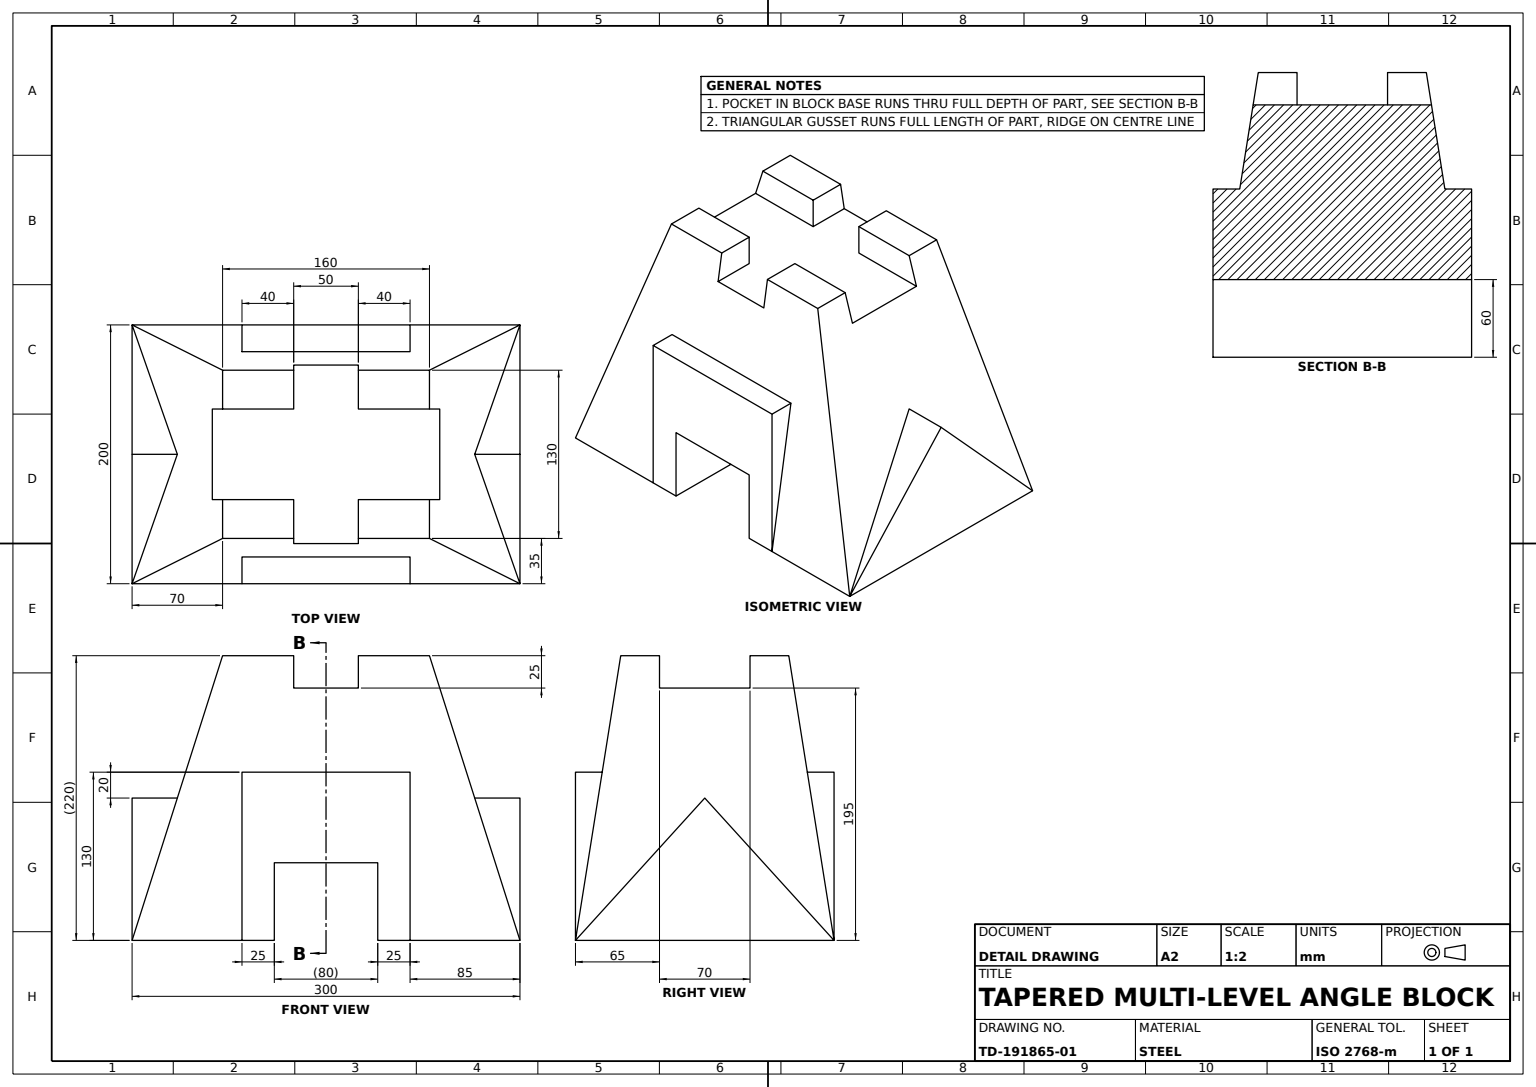
ISO-10303-21;
HEADER;
FILE_DESCRIPTION((''),'2;1');
FILE_NAME('','',(''),(''),'','','');
FILE_SCHEMA(('AUTOMOTIVE_DESIGN'));
ENDSEC;
DATA;
#1=APPLICATION_CONTEXT('');
#2=PRODUCT_CONTEXT('',#1,'mechanical');
#3=PRODUCT('','','',(#2));
#4=PRODUCT_DEFINITION_FORMATION('','',#3);
#5=PRODUCT_DEFINITION_CONTEXT('',#1,'design');
#6=PRODUCT_DEFINITION('','',#4,#5);
#7=PRODUCT_DEFINITION_SHAPE('','',#6);
#8=(LENGTH_UNIT()NAMED_UNIT(*)SI_UNIT(.MILLI.,.METRE.));
#9=(NAMED_UNIT(*)PLANE_ANGLE_UNIT()SI_UNIT($,.RADIAN.));
#10=(NAMED_UNIT(*)SI_UNIT($,.STERADIAN.)SOLID_ANGLE_UNIT());
#11=UNCERTAINTY_MEASURE_WITH_UNIT(LENGTH_MEASURE(0.005),#8,'distance_accuracy_value','');
#12=(GEOMETRIC_REPRESENTATION_CONTEXT(3)GLOBAL_UNCERTAINTY_ASSIGNED_CONTEXT((#11))GLOBAL_UNIT_ASSIGNED_CONTEXT((#8,#9,#10))REPRESENTATION_CONTEXT('',''));
#13=CARTESIAN_POINT('',(-100.,65.,130.));
#14=VERTEX_POINT('',#13);
#15=CARTESIAN_POINT('',(-100.,65.,0.));
#16=VERTEX_POINT('',#15);
#17=DIRECTION('',(0.,0.,-1.));
#18=VECTOR('',#17,1000.);
#19=LINE('',#13,#18);
#20=EDGE_CURVE('',#14,#16,#19,.T.);
#21=ORIENTED_EDGE('',*,*,#20,.T.);
#22=CARTESIAN_POINT('',(-100.,40.,0.));
#23=VERTEX_POINT('',#22);
#24=DIRECTION('',(0.,-1.,0.));
#25=VECTOR('',#24,1000.);
#26=LINE('',#15,#25);
#27=EDGE_CURVE('',#16,#23,#26,.T.);
#28=ORIENTED_EDGE('',*,*,#27,.T.);
#29=CARTESIAN_POINT('',(-100.,40.,60.));
#30=VERTEX_POINT('',#29);
#31=LINE('',#22,#18);
#32=EDGE_CURVE('',#30,#23,#31,.T.);
#33=ORIENTED_EDGE('',*,*,#32,.F.);
#34=CARTESIAN_POINT('',(-100.,-40.,60.));
#35=VERTEX_POINT('',#34);
#36=CARTESIAN_POINT('',(-100.,0.,60.));
#37=DIRECTION('',(0.,1.,0.));
#38=VECTOR('',#37,1000.);
#39=LINE('',#36,#38);
#40=EDGE_CURVE('',#35,#30,#39,.T.);
#41=ORIENTED_EDGE('',*,*,#40,.F.);
#42=CARTESIAN_POINT('',(-100.,-40.,0.));
#43=VERTEX_POINT('',#42);
#44=DIRECTION('',(0.,0.,1.));
#45=VECTOR('',#44,1000.);
#46=LINE('',#42,#45);
#47=EDGE_CURVE('',#43,#35,#46,.T.);
#48=ORIENTED_EDGE('',*,*,#47,.F.);
#49=CARTESIAN_POINT('',(-100.,-65.,0.));
#50=VERTEX_POINT('',#49);
#51=EDGE_CURVE('',#43,#50,#26,.T.);
#52=ORIENTED_EDGE('',*,*,#51,.T.);
#53=CARTESIAN_POINT('',(-100.,-65.,130.));
#54=VERTEX_POINT('',#53);
#55=LINE('',#49,#45);
#56=EDGE_CURVE('',#50,#54,#55,.T.);
#57=ORIENTED_EDGE('',*,*,#56,.T.);
#58=LINE('',#53,#38);
#59=EDGE_CURVE('',#54,#14,#58,.T.);
#60=ORIENTED_EDGE('',*,*,#59,.T.);
#61=EDGE_LOOP('',(#21,#28,#33,#41,#48,#52,#57,#60));
#62=FACE_BOUND('',#61,.T.);
#63=CARTESIAN_POINT('',(-100.,0.,0.));
#64=DIRECTION('',(-1.,0.,0.));
#65=AXIS2_PLACEMENT_3D('',#63,#64,#44);
#66=PLANE('',#65);
#67=ADVANCED_FACE('',(#62),#66,.T.);
#68=CARTESIAN_POINT('',(100.,150.,0.));
#69=VERTEX_POINT('',#68);
#70=CARTESIAN_POINT('',(0.,150.,110.));
#71=VERTEX_POINT('',#70);
#72=DIRECTION('',(-0.672672794,0.,0.739940073));
#73=VECTOR('',#72,1000.);
#74=LINE('',#68,#73);
#75=EDGE_CURVE('',#69,#71,#74,.T.);
#76=ORIENTED_EDGE('',*,*,#75,.F.);
#77=CARTESIAN_POINT('',(-100.,150.,0.));
#78=VERTEX_POINT('',#77);
#79=VECTOR('',#64,1000.);
#80=LINE('',#68,#79);
#81=EDGE_CURVE('',#69,#78,#80,.T.);
#82=ORIENTED_EDGE('',*,*,#81,.T.);
#83=DIRECTION('',(-0.672672794,0.,-0.739940073));
#84=VECTOR('',#83,1000.);
#85=LINE('',#70,#84);
#86=EDGE_CURVE('',#71,#78,#85,.T.);
#87=ORIENTED_EDGE('',*,*,#86,.F.);
#88=EDGE_LOOP('',(#76,#82,#87));
#89=FACE_BOUND('',#88,.T.);
#90=CARTESIAN_POINT('',(0.,150.,0.));
#91=AXIS2_PLACEMENT_3D('',#90,#24,#17);
#92=PLANE('',#91);
#93=ADVANCED_FACE('',(#89),#92,.F.);
#94=CARTESIAN_POINT('',(35.,-25.,195.));
#95=VERTEX_POINT('',#94);
#96=CARTESIAN_POINT('',(35.,-25.,220.));
#97=VERTEX_POINT('',#96);
#98=CARTESIAN_POINT('',(35.,-25.,265.));
#99=LINE('',#98,#18);
#100=EDGE_CURVE('',#95,#97,#99,.F.);
#101=ORIENTED_EDGE('',*,*,#100,.F.);
#102=CARTESIAN_POINT('',(35.,-87.954545,195.));
#103=VERTEX_POINT('',#102);
#104=CARTESIAN_POINT('',(35.,-220.,195.));
#105=LINE('',#104,#38);
#106=EDGE_CURVE('',#103,#95,#105,.T.);
#107=ORIENTED_EDGE('',*,*,#106,.F.);
#108=CARTESIAN_POINT('',(35.,-80.,220.));
#109=VERTEX_POINT('',#108);
#110=DIRECTION('',(0.,-0.303203657,-0.95292578));
#111=VECTOR('',#110,1000.);
#112=LINE('',#108,#111);
#113=EDGE_CURVE('',#109,#103,#112,.T.);
#114=ORIENTED_EDGE('',*,*,#113,.F.);
#115=CARTESIAN_POINT('',(35.,-220.,220.));
#116=LINE('',#115,#38);
#117=EDGE_CURVE('',#109,#97,#116,.T.);
#118=ORIENTED_EDGE('',*,*,#117,.T.);
#119=EDGE_LOOP('',(#101,#107,#114,#118));
#120=FACE_BOUND('',#119,.T.);
#121=DIRECTION('',(1.,0.,0.));
#122=AXIS2_PLACEMENT_3D('',#115,#121,#17);
#123=PLANE('',#122);
#124=ADVANCED_FACE('',(#120),#123,.F.);
#125=ORIENTED_EDGE('',*,*,#47,.T.);
#126=CARTESIAN_POINT('',(100.,-40.,60.));
#127=VERTEX_POINT('',#126);
#128=CARTESIAN_POINT('',(145.,-40.,60.));
#129=LINE('',#128,#79);
#130=EDGE_CURVE('',#35,#127,#129,.F.);
#131=ORIENTED_EDGE('',*,*,#130,.T.);
#132=CARTESIAN_POINT('',(100.,-40.,0.));
#133=VERTEX_POINT('',#132);
#134=LINE('',#132,#45);
#135=EDGE_CURVE('',#133,#127,#134,.T.);
#136=ORIENTED_EDGE('',*,*,#135,.F.);
#137=CARTESIAN_POINT('',(145.,-40.,0.));
#138=LINE('',#137,#79);
#139=EDGE_CURVE('',#133,#43,#138,.T.);
#140=ORIENTED_EDGE('',*,*,#139,.T.);
#141=EDGE_LOOP('',(#125,#131,#136,#140));
#142=FACE_BOUND('',#141,.T.);
#143=AXIS2_PLACEMENT_3D('',#137,#24,#17);
#144=PLANE('',#143);
#145=ADVANCED_FACE('',(#142),#144,.F.);
#146=CARTESIAN_POINT('',(-35.,-25.,195.));
#147=VERTEX_POINT('',#146);
#148=CARTESIAN_POINT('',(-35.,-25.,220.));
#149=VERTEX_POINT('',#148);
#150=CARTESIAN_POINT('',(-35.,-25.,265.));
#151=LINE('',#150,#18);
#152=EDGE_CURVE('',#147,#149,#151,.F.);
#153=ORIENTED_EDGE('',*,*,#152,.F.);
#154=CARTESIAN_POINT('',(-68.977273,-25.,195.));
#155=VERTEX_POINT('',#154);
#156=CARTESIAN_POINT('',(-70.,-25.,195.));
#157=VECTOR('',#121,1000.);
#158=LINE('',#156,#157);
#159=EDGE_CURVE('',#147,#155,#158,.F.);
#160=ORIENTED_EDGE('',*,*,#159,.T.);
#161=CARTESIAN_POINT('',(-65.,-25.,220.));
#162=VERTEX_POINT('',#161);
#163=CARTESIAN_POINT('',(-100.,-25.,0.));
#164=DIRECTION('',(-0.157115049,0.,-0.987580306));
#165=VECTOR('',#164,1000.);
#166=LINE('',#163,#165);
#167=EDGE_CURVE('',#162,#155,#166,.T.);
#168=ORIENTED_EDGE('',*,*,#167,.F.);
#169=CARTESIAN_POINT('',(100.,-25.,220.));
#170=LINE('',#169,#157);
#171=EDGE_CURVE('',#162,#149,#170,.T.);
#172=ORIENTED_EDGE('',*,*,#171,.T.);
#173=EDGE_LOOP('',(#153,#160,#168,#172));
#174=FACE_BOUND('',#173,.T.);
#175=CARTESIAN_POINT('',(-70.,-25.,265.));
#176=AXIS2_PLACEMENT_3D('',#175,#37,#64);
#177=PLANE('',#176);
#178=ADVANCED_FACE('',(#174),#177,.T.);
#179=CARTESIAN_POINT('',(-35.,-80.,220.));
#180=VERTEX_POINT('',#179);
#181=CARTESIAN_POINT('',(-35.,-220.,220.));
#182=LINE('',#181,#38);
#183=EDGE_CURVE('',#180,#149,#182,.T.);
#184=ORIENTED_EDGE('',*,*,#183,.F.);
#185=CARTESIAN_POINT('',(-35.,-87.954545,195.));
#186=VERTEX_POINT('',#185);
#187=DIRECTION('',(0.,0.303203657,0.95292578));
#188=VECTOR('',#187,1000.);
#189=LINE('',#179,#188);
#190=EDGE_CURVE('',#186,#180,#189,.T.);
#191=ORIENTED_EDGE('',*,*,#190,.F.);
#192=CARTESIAN_POINT('',(-35.,-220.,195.));
#193=LINE('',#192,#38);
#194=EDGE_CURVE('',#186,#147,#193,.T.);
#195=ORIENTED_EDGE('',*,*,#194,.T.);
#196=ORIENTED_EDGE('',*,*,#152,.T.);
#197=EDGE_LOOP('',(#184,#191,#195,#196));
#198=FACE_BOUND('',#197,.T.);
#199=AXIS2_PLACEMENT_3D('',#192,#64,#44);
#200=PLANE('',#199);
#201=ADVANCED_FACE('',(#198),#200,.F.);
#202=ORIENTED_EDGE('',*,*,#40,.T.);
#203=CARTESIAN_POINT('',(100.,40.,60.));
#204=VERTEX_POINT('',#203);
#205=CARTESIAN_POINT('',(145.,40.,60.));
#206=LINE('',#205,#79);
#207=EDGE_CURVE('',#30,#204,#206,.F.);
#208=ORIENTED_EDGE('',*,*,#207,.T.);
#209=CARTESIAN_POINT('',(100.,0.,60.));
#210=LINE('',#209,#38);
#211=EDGE_CURVE('',#127,#204,#210,.T.);
#212=ORIENTED_EDGE('',*,*,#211,.F.);
#213=ORIENTED_EDGE('',*,*,#130,.F.);
#214=EDGE_LOOP('',(#202,#208,#212,#213));
#215=FACE_BOUND('',#214,.T.);
#216=AXIS2_PLACEMENT_3D('',#128,#44,#121);
#217=PLANE('',#216);
#218=ADVANCED_FACE('',(#215),#217,.F.);
#219=CARTESIAN_POINT('',(65.,-25.,220.));
#220=VERTEX_POINT('',#219);
#221=LINE('',#169,#79);
#222=EDGE_CURVE('',#220,#97,#221,.T.);
#223=ORIENTED_EDGE('',*,*,#222,.F.);
#224=CARTESIAN_POINT('',(68.977273,-25.,195.));
#225=VERTEX_POINT('',#224);
#226=DIRECTION('',(0.157115049,0.,-0.987580306));
#227=VECTOR('',#226,1000.);
#228=LINE('',#219,#227);
#229=EDGE_CURVE('',#220,#225,#228,.T.);
#230=ORIENTED_EDGE('',*,*,#229,.T.);
#231=CARTESIAN_POINT('',(70.,-25.,195.));
#232=LINE('',#231,#79);
#233=EDGE_CURVE('',#95,#225,#232,.F.);
#234=ORIENTED_EDGE('',*,*,#233,.F.);
#235=ORIENTED_EDGE('',*,*,#100,.T.);
#236=EDGE_LOOP('',(#223,#230,#234,#235));
#237=FACE_BOUND('',#236,.T.);
#238=CARTESIAN_POINT('',(70.,-25.,265.));
#239=AXIS2_PLACEMENT_3D('',#238,#24,#121);
#240=PLANE('',#239);
#241=ADVANCED_FACE('',(#237),#240,.F.);
#242=CARTESIAN_POINT('',(100.,65.,0.));
#243=VERTEX_POINT('',#242);
#244=CARTESIAN_POINT('',(79.318182,65.,130.));
#245=VERTEX_POINT('',#244);
#246=CARTESIAN_POINT('',(65.,65.,220.));
#247=DIRECTION('',(-0.157115049,0.,0.987580306));
#248=VECTOR('',#247,1000.);
#249=LINE('',#246,#248);
#250=EDGE_CURVE('',#243,#245,#249,.T.);
#251=ORIENTED_EDGE('',*,*,#250,.T.);
#252=CARTESIAN_POINT('',(100.,65.,130.));
#253=VERTEX_POINT('',#252);
#254=LINE('',#252,#79);
#255=EDGE_CURVE('',#253,#245,#254,.T.);
#256=ORIENTED_EDGE('',*,*,#255,.F.);
#257=LINE('',#252,#18);
#258=EDGE_CURVE('',#253,#243,#257,.T.);
#259=ORIENTED_EDGE('',*,*,#258,.T.);
#260=EDGE_LOOP('',(#251,#256,#259));
#261=FACE_BOUND('',#260,.T.);
#262=AXIS2_PLACEMENT_3D('',#252,#37,#44);
#263=PLANE('',#262);
#264=ADVANCED_FACE('',(#261),#263,.T.);
#265=CARTESIAN_POINT('',(0.,115.,110.));
#266=VERTEX_POINT('',#265);
#267=CARTESIAN_POINT('',(-14.255091,119.989282,94.3194));
#268=DIRECTION('',(0.654770604,-0.229169712,0.720247665));
#269=VECTOR('',#268,1000.);
#270=LINE('',#267,#269);
#271=EDGE_CURVE('',#78,#266,#270,.T.);
#272=ORIENTED_EDGE('',*,*,#271,.F.);
#273=CARTESIAN_POINT('',(-65.,80.,220.));
#274=VERTEX_POINT('',#273);
#275=CARTESIAN_POINT('',(-95.506648,141.013297,28.243925));
#276=DIRECTION('',(-0.149889154,0.299778307,-0.942160394));
#277=VECTOR('',#276,1000.);
#278=LINE('',#275,#277);
#279=EDGE_CURVE('',#78,#274,#278,.F.);
#280=ORIENTED_EDGE('',*,*,#279,.T.);
#281=CARTESIAN_POINT('',(-35.,80.,220.));
#282=VERTEX_POINT('',#281);
#283=CARTESIAN_POINT('',(100.,80.,220.));
#284=LINE('',#283,#79);
#285=EDGE_CURVE('',#282,#274,#284,.T.);
#286=ORIENTED_EDGE('',*,*,#285,.F.);
#287=CARTESIAN_POINT('',(-35.,87.954545,195.));
#288=VERTEX_POINT('',#287);
#289=CARTESIAN_POINT('',(-35.,150.,0.));
#290=DIRECTION('',(0.,0.303203657,-0.95292578));
#291=VECTOR('',#290,1000.);
#292=LINE('',#289,#291);
#293=EDGE_CURVE('',#282,#288,#292,.T.);
#294=ORIENTED_EDGE('',*,*,#293,.T.);
#295=CARTESIAN_POINT('',(35.,87.954545,195.));
#296=VERTEX_POINT('',#295);
#297=CARTESIAN_POINT('',(100.,87.954545,195.));
#298=LINE('',#297,#157);
#299=EDGE_CURVE('',#288,#296,#298,.T.);
#300=ORIENTED_EDGE('',*,*,#299,.T.);
#301=CARTESIAN_POINT('',(35.,80.,220.));
#302=VERTEX_POINT('',#301);
#303=CARTESIAN_POINT('',(35.,150.,0.));
#304=DIRECTION('',(0.,-0.303203657,0.95292578));
#305=VECTOR('',#304,1000.);
#306=LINE('',#303,#305);
#307=EDGE_CURVE('',#296,#302,#306,.T.);
#308=ORIENTED_EDGE('',*,*,#307,.T.);
#309=CARTESIAN_POINT('',(65.,80.,220.));
#310=VERTEX_POINT('',#309);
#311=EDGE_CURVE('',#310,#302,#284,.T.);
#312=ORIENTED_EDGE('',*,*,#311,.F.);
#313=DIRECTION('',(-0.149889154,-0.299778307,0.942160394));
#314=VECTOR('',#313,1000.);
#315=LINE('',#68,#314);
#316=EDGE_CURVE('',#310,#69,#315,.F.);
#317=ORIENTED_EDGE('',*,*,#316,.T.);
#318=DIRECTION('',(0.654770604,0.229169712,-0.720247665));
#319=VECTOR('',#318,1000.);
#320=LINE('',#68,#319);
#321=EDGE_CURVE('',#266,#69,#320,.T.);
#322=ORIENTED_EDGE('',*,*,#321,.F.);
#323=EDGE_LOOP('',(#272,#280,#286,#294,#300,#308,#312,#317,#322));
#324=FACE_BOUND('',#323,.T.);
#325=DIRECTION('',(0.,-0.95292578,-0.303203657));
#326=AXIS2_PLACEMENT_3D('',#68,#325,#290);
#327=PLANE('',#326);
#328=ADVANCED_FACE('',(#324),#327,.F.);
#329=CARTESIAN_POINT('',(65.,-80.,220.));
#330=VERTEX_POINT('',#329);
#331=CARTESIAN_POINT('',(100.,-80.,220.));
#332=LINE('',#331,#79);
#333=EDGE_CURVE('',#330,#109,#332,.T.);
#334=ORIENTED_EDGE('',*,*,#333,.T.);
#335=ORIENTED_EDGE('',*,*,#113,.T.);
#336=CARTESIAN_POINT('',(100.,-87.954545,195.));
#337=LINE('',#336,#79);
#338=EDGE_CURVE('',#103,#186,#337,.T.);
#339=ORIENTED_EDGE('',*,*,#338,.T.);
#340=ORIENTED_EDGE('',*,*,#190,.T.);
#341=CARTESIAN_POINT('',(-65.,-80.,220.));
#342=VERTEX_POINT('',#341);
#343=EDGE_CURVE('',#180,#342,#332,.T.);
#344=ORIENTED_EDGE('',*,*,#343,.T.);
#345=CARTESIAN_POINT('',(-100.,-150.,0.));
#346=VERTEX_POINT('',#345);
#347=CARTESIAN_POINT('',(-61.292985,-72.58597,243.301238));
#348=DIRECTION('',(0.149889154,0.299778307,0.942160394));
#349=VECTOR('',#348,1000.);
#350=LINE('',#347,#349);
#351=EDGE_CURVE('',#342,#346,#350,.F.);
#352=ORIENTED_EDGE('',*,*,#351,.T.);
#353=CARTESIAN_POINT('',(0.,-115.,110.));
#354=VERTEX_POINT('',#353);
#355=DIRECTION('',(-0.654770604,-0.229169712,-0.720247665));
#356=VECTOR('',#355,1000.);
#357=LINE('',#331,#356);
#358=EDGE_CURVE('',#354,#346,#357,.T.);
#359=ORIENTED_EDGE('',*,*,#358,.F.);
#360=CARTESIAN_POINT('',(100.,-150.,0.));
#361=VERTEX_POINT('',#360);
#362=CARTESIAN_POINT('',(-14.255091,-110.010718,125.6806));
#363=DIRECTION('',(-0.654770604,0.229169712,0.720247665));
#364=VECTOR('',#363,1000.);
#365=LINE('',#362,#364);
#366=EDGE_CURVE('',#361,#354,#365,.T.);
#367=ORIENTED_EDGE('',*,*,#366,.F.);
#368=CARTESIAN_POINT('',(65.786337,-81.572673,215.057313));
#369=DIRECTION('',(0.149889154,-0.299778307,-0.942160394));
#370=VECTOR('',#369,1000.);
#371=LINE('',#368,#370);
#372=EDGE_CURVE('',#361,#330,#371,.F.);
#373=ORIENTED_EDGE('',*,*,#372,.T.);
#374=EDGE_LOOP('',(#334,#335,#339,#340,#344,#352,#359,#367,#373));
#375=FACE_BOUND('',#374,.T.);
#376=DIRECTION('',(0.,0.95292578,-0.303203657));
#377=AXIS2_PLACEMENT_3D('',#331,#376,#187);
#378=PLANE('',#377);
#379=ADVANCED_FACE('',(#375),#378,.F.);
#380=CARTESIAN_POINT('',(35.,25.,220.));
#381=VERTEX_POINT('',#380);
#382=CARTESIAN_POINT('',(65.,25.,220.));
#383=VERTEX_POINT('',#382);
#384=CARTESIAN_POINT('',(100.,25.,220.));
#385=LINE('',#384,#157);
#386=EDGE_CURVE('',#381,#383,#385,.T.);
#387=ORIENTED_EDGE('',*,*,#386,.T.);
#388=CARTESIAN_POINT('',(65.,-250.,220.));
#389=LINE('',#388,#38);
#390=EDGE_CURVE('',#383,#310,#389,.T.);
#391=ORIENTED_EDGE('',*,*,#390,.T.);
#392=ORIENTED_EDGE('',*,*,#311,.T.);
#393=EDGE_CURVE('',#381,#302,#116,.T.);
#394=ORIENTED_EDGE('',*,*,#393,.F.);
#395=EDGE_LOOP('',(#387,#391,#392,#394));
#396=FACE_BOUND('',#395,.T.);
#397=AXIS2_PLACEMENT_3D('',#283,#17,#64);
#398=PLANE('',#397);
#399=ADVANCED_FACE('',(#396),#398,.F.);
#400=CARTESIAN_POINT('',(100.,-65.,0.));
#401=VERTEX_POINT('',#400);
#402=CARTESIAN_POINT('',(100.,-65.,130.));
#403=VERTEX_POINT('',#402);
#404=LINE('',#400,#45);
#405=EDGE_CURVE('',#401,#403,#404,.T.);
#406=ORIENTED_EDGE('',*,*,#405,.T.);
#407=CARTESIAN_POINT('',(79.318182,-65.,130.));
#408=VERTEX_POINT('',#407);
#409=LINE('',#402,#79);
#410=EDGE_CURVE('',#403,#408,#409,.T.);
#411=ORIENTED_EDGE('',*,*,#410,.T.);
#412=CARTESIAN_POINT('',(65.,-65.,220.));
#413=LINE('',#412,#227);
#414=EDGE_CURVE('',#408,#401,#413,.T.);
#415=ORIENTED_EDGE('',*,*,#414,.T.);
#416=EDGE_LOOP('',(#406,#411,#415));
#417=FACE_BOUND('',#416,.T.);
#418=AXIS2_PLACEMENT_3D('',#400,#24,#17);
#419=PLANE('',#418);
#420=ADVANCED_FACE('',(#417),#419,.T.);
#421=CARTESIAN_POINT('',(-35.,25.,220.));
#422=VERTEX_POINT('',#421);
#423=EDGE_CURVE('',#422,#282,#182,.T.);
#424=ORIENTED_EDGE('',*,*,#423,.F.);
#425=CARTESIAN_POINT('',(-35.,25.,195.));
#426=VERTEX_POINT('',#425);
#427=CARTESIAN_POINT('',(-35.,25.,265.));
#428=LINE('',#427,#18);
#429=EDGE_CURVE('',#426,#422,#428,.F.);
#430=ORIENTED_EDGE('',*,*,#429,.F.);
#431=EDGE_CURVE('',#426,#288,#193,.T.);
#432=ORIENTED_EDGE('',*,*,#431,.T.);
#433=ORIENTED_EDGE('',*,*,#293,.F.);
#434=EDGE_LOOP('',(#424,#430,#432,#433));
#435=FACE_BOUND('',#434,.T.);
#436=ADVANCED_FACE('',(#435),#200,.F.);
#437=ORIENTED_EDGE('',*,*,#167,.T.);
#438=CARTESIAN_POINT('',(-68.977273,25.,195.));
#439=VERTEX_POINT('',#438);
#440=CARTESIAN_POINT('',(-68.977273,-250.,195.));
#441=LINE('',#440,#38);
#442=EDGE_CURVE('',#155,#439,#441,.T.);
#443=ORIENTED_EDGE('',*,*,#442,.T.);
#444=CARTESIAN_POINT('',(-65.,25.,220.));
#445=VERTEX_POINT('',#444);
#446=CARTESIAN_POINT('',(-100.,25.,0.));
#447=DIRECTION('',(0.157115049,0.,0.987580306));
#448=VECTOR('',#447,1000.);
#449=LINE('',#446,#448);
#450=EDGE_CURVE('',#439,#445,#449,.T.);
#451=ORIENTED_EDGE('',*,*,#450,.T.);
#452=CARTESIAN_POINT('',(-65.,-250.,220.));
#453=LINE('',#452,#38);
#454=EDGE_CURVE('',#445,#274,#453,.T.);
#455=ORIENTED_EDGE('',*,*,#454,.T.);
#456=ORIENTED_EDGE('',*,*,#279,.F.);
#457=LINE('',#345,#38);
#458=EDGE_CURVE('',#16,#78,#457,.T.);
#459=ORIENTED_EDGE('',*,*,#458,.F.);
#460=CARTESIAN_POINT('',(-79.318182,65.,130.));
#461=VERTEX_POINT('',#460);
#462=LINE('',#15,#165);
#463=EDGE_CURVE('',#461,#16,#462,.T.);
#464=ORIENTED_EDGE('',*,*,#463,.F.);
#465=CARTESIAN_POINT('',(-79.318182,-65.,130.));
#466=VERTEX_POINT('',#465);
#467=CARTESIAN_POINT('',(-79.318182,-250.,130.));
#468=LINE('',#467,#38);
#469=EDGE_CURVE('',#466,#461,#468,.T.);
#470=ORIENTED_EDGE('',*,*,#469,.F.);
#471=LINE('',#49,#448);
#472=EDGE_CURVE('',#50,#466,#471,.T.);
#473=ORIENTED_EDGE('',*,*,#472,.F.);
#474=EDGE_CURVE('',#346,#50,#457,.T.);
#475=ORIENTED_EDGE('',*,*,#474,.F.);
#476=ORIENTED_EDGE('',*,*,#351,.F.);
#477=EDGE_CURVE('',#342,#162,#453,.T.);
#478=ORIENTED_EDGE('',*,*,#477,.T.);
#479=EDGE_LOOP('',(#437,#443,#451,#455,#456,#459,#464,#470,#473,#475,#476,#478));
#480=FACE_BOUND('',#479,.T.);
#481=CARTESIAN_POINT('',(-100.,-250.,0.));
#482=DIRECTION('',(-0.987580306,0.,0.157115049));
#483=AXIS2_PLACEMENT_3D('',#481,#482,#447);
#484=PLANE('',#483);
#485=ADVANCED_FACE('',(#480),#484,.T.);
#486=ORIENTED_EDGE('',*,*,#472,.T.);
#487=EDGE_CURVE('',#466,#54,#409,.T.);
#488=ORIENTED_EDGE('',*,*,#487,.T.);
#489=ORIENTED_EDGE('',*,*,#56,.F.);
#490=EDGE_LOOP('',(#486,#488,#489));
#491=FACE_BOUND('',#490,.T.);
#492=ADVANCED_FACE('',(#491),#419,.T.);
#493=CARTESIAN_POINT('',(68.977273,25.,195.));
#494=VERTEX_POINT('',#493);
#495=LINE('',#382,#248);
#496=EDGE_CURVE('',#494,#383,#495,.T.);
#497=ORIENTED_EDGE('',*,*,#496,.F.);
#498=CARTESIAN_POINT('',(68.977273,-250.,195.));
#499=LINE('',#498,#38);
#500=EDGE_CURVE('',#225,#494,#499,.T.);
#501=ORIENTED_EDGE('',*,*,#500,.F.);
#502=ORIENTED_EDGE('',*,*,#229,.F.);
#503=EDGE_CURVE('',#330,#220,#389,.T.);
#504=ORIENTED_EDGE('',*,*,#503,.F.);
#505=ORIENTED_EDGE('',*,*,#372,.F.);
#506=LINE('',#360,#38);
#507=EDGE_CURVE('',#361,#401,#506,.T.);
#508=ORIENTED_EDGE('',*,*,#507,.T.);
#509=ORIENTED_EDGE('',*,*,#414,.F.);
#510=CARTESIAN_POINT('',(79.318182,-250.,130.));
#511=LINE('',#510,#25);
#512=EDGE_CURVE('',#245,#408,#511,.T.);
#513=ORIENTED_EDGE('',*,*,#512,.F.);
#514=ORIENTED_EDGE('',*,*,#250,.F.);
#515=EDGE_CURVE('',#243,#69,#506,.T.);
#516=ORIENTED_EDGE('',*,*,#515,.T.);
#517=ORIENTED_EDGE('',*,*,#316,.F.);
#518=ORIENTED_EDGE('',*,*,#390,.F.);
#519=EDGE_LOOP('',(#497,#501,#502,#504,#505,#508,#509,#513,#514,#516,#517,#518));
#520=FACE_BOUND('',#519,.T.);
#521=DIRECTION('',(0.987580306,0.,0.157115049));
#522=AXIS2_PLACEMENT_3D('',#388,#521,#226);
#523=PLANE('',#522);
#524=ADVANCED_FACE('',(#520),#523,.T.);
#525=ORIENTED_EDGE('',*,*,#423,.T.);
#526=ORIENTED_EDGE('',*,*,#285,.T.);
#527=ORIENTED_EDGE('',*,*,#454,.F.);
#528=LINE('',#384,#79);
#529=EDGE_CURVE('',#422,#445,#528,.T.);
#530=ORIENTED_EDGE('',*,*,#529,.F.);
#531=EDGE_LOOP('',(#525,#526,#527,#530));
#532=FACE_BOUND('',#531,.T.);
#533=ADVANCED_FACE('',(#532),#398,.F.);
#534=CARTESIAN_POINT('',(100.,40.,0.));
#535=VERTEX_POINT('',#534);
#536=CARTESIAN_POINT('',(145.,40.,0.));
#537=LINE('',#536,#79);
#538=EDGE_CURVE('',#535,#23,#537,.T.);
#539=ORIENTED_EDGE('',*,*,#538,.T.);
#540=ORIENTED_EDGE('',*,*,#27,.F.);
#541=ORIENTED_EDGE('',*,*,#458,.T.);
#542=ORIENTED_EDGE('',*,*,#81,.F.);
#543=ORIENTED_EDGE('',*,*,#515,.F.);
#544=LINE('',#242,#25);
#545=EDGE_CURVE('',#243,#535,#544,.T.);
#546=ORIENTED_EDGE('',*,*,#545,.T.);
#547=EDGE_LOOP('',(#539,#540,#541,#542,#543,#546));
#548=FACE_BOUND('',#547,.T.);
#549=AXIS2_PLACEMENT_3D('',#360,#44,#121);
#550=PLANE('',#549);
#551=ADVANCED_FACE('',(#548),#550,.F.);
#552=CARTESIAN_POINT('',(0.,-150.,110.));
#553=VERTEX_POINT('',#552);
#554=LINE('',#552,#38);
#555=EDGE_CURVE('',#553,#354,#554,.T.);
#556=ORIENTED_EDGE('',*,*,#555,.T.);
#557=ORIENTED_EDGE('',*,*,#358,.T.);
#558=LINE('',#552,#84);
#559=EDGE_CURVE('',#553,#346,#558,.T.);
#560=ORIENTED_EDGE('',*,*,#559,.F.);
#561=EDGE_LOOP('',(#556,#557,#560));
#562=FACE_BOUND('',#561,.T.);
#563=DIRECTION('',(0.739940073,0.,-0.672672794));
#564=AXIS2_PLACEMENT_3D('',#552,#563,#83);
#565=PLANE('',#564);
#566=ADVANCED_FACE('',(#562),#565,.F.);
#567=ORIENTED_EDGE('',*,*,#20,.F.);
#568=EDGE_CURVE('',#461,#14,#254,.T.);
#569=ORIENTED_EDGE('',*,*,#568,.F.);
#570=ORIENTED_EDGE('',*,*,#463,.T.);
#571=EDGE_LOOP('',(#567,#569,#570));
#572=FACE_BOUND('',#571,.T.);
#573=ADVANCED_FACE('',(#572),#263,.T.);
#574=ORIENTED_EDGE('',*,*,#211,.T.);
#575=LINE('',#534,#18);
#576=EDGE_CURVE('',#204,#535,#575,.T.);
#577=ORIENTED_EDGE('',*,*,#576,.T.);
#578=ORIENTED_EDGE('',*,*,#545,.F.);
#579=ORIENTED_EDGE('',*,*,#258,.F.);
#580=LINE('',#402,#38);
#581=EDGE_CURVE('',#403,#253,#580,.T.);
#582=ORIENTED_EDGE('',*,*,#581,.F.);
#583=ORIENTED_EDGE('',*,*,#405,.F.);
#584=EDGE_CURVE('',#133,#401,#544,.T.);
#585=ORIENTED_EDGE('',*,*,#584,.F.);
#586=ORIENTED_EDGE('',*,*,#135,.T.);
#587=EDGE_LOOP('',(#574,#577,#578,#579,#582,#583,#585,#586));
#588=FACE_BOUND('',#587,.T.);
#589=CARTESIAN_POINT('',(100.,0.,0.));
#590=AXIS2_PLACEMENT_3D('',#589,#64,#44);
#591=PLANE('',#590);
#592=ADVANCED_FACE('',(#588),#591,.F.);
#593=ORIENTED_EDGE('',*,*,#207,.F.);
#594=ORIENTED_EDGE('',*,*,#32,.T.);
#595=ORIENTED_EDGE('',*,*,#538,.F.);
#596=ORIENTED_EDGE('',*,*,#576,.F.);
#597=EDGE_LOOP('',(#593,#594,#595,#596));
#598=FACE_BOUND('',#597,.T.);
#599=AXIS2_PLACEMENT_3D('',#205,#37,#44);
#600=PLANE('',#599);
#601=ADVANCED_FACE('',(#598),#600,.F.);
#602=LINE('',#425,#79);
#603=EDGE_CURVE('',#439,#426,#602,.F.);
#604=ORIENTED_EDGE('',*,*,#603,.T.);
#605=ORIENTED_EDGE('',*,*,#429,.T.);
#606=ORIENTED_EDGE('',*,*,#529,.T.);
#607=ORIENTED_EDGE('',*,*,#450,.F.);
#608=EDGE_LOOP('',(#604,#605,#606,#607));
#609=FACE_BOUND('',#608,.T.);
#610=AXIS2_PLACEMENT_3D('',#427,#24,#121);
#611=PLANE('',#610);
#612=ADVANCED_FACE('',(#609),#611,.T.);
#613=ORIENTED_EDGE('',*,*,#386,.F.);
#614=CARTESIAN_POINT('',(35.,25.,195.));
#615=VERTEX_POINT('',#614);
#616=CARTESIAN_POINT('',(35.,25.,265.));
#617=LINE('',#616,#18);
#618=EDGE_CURVE('',#615,#381,#617,.F.);
#619=ORIENTED_EDGE('',*,*,#618,.F.);
#620=LINE('',#614,#157);
#621=EDGE_CURVE('',#494,#615,#620,.F.);
#622=ORIENTED_EDGE('',*,*,#621,.F.);
#623=ORIENTED_EDGE('',*,*,#496,.T.);
#624=EDGE_LOOP('',(#613,#619,#622,#623));
#625=FACE_BOUND('',#624,.T.);
#626=AXIS2_PLACEMENT_3D('',#616,#37,#64);
#627=PLANE('',#626);
#628=ADVANCED_FACE('',(#625),#627,.F.);
#629=ORIENTED_EDGE('',*,*,#442,.F.);
#630=ORIENTED_EDGE('',*,*,#159,.F.);
#631=ORIENTED_EDGE('',*,*,#194,.F.);
#632=ORIENTED_EDGE('',*,*,#338,.F.);
#633=ORIENTED_EDGE('',*,*,#106,.T.);
#634=ORIENTED_EDGE('',*,*,#233,.T.);
#635=ORIENTED_EDGE('',*,*,#500,.T.);
#636=ORIENTED_EDGE('',*,*,#621,.T.);
#637=EDGE_CURVE('',#615,#296,#105,.T.);
#638=ORIENTED_EDGE('',*,*,#637,.T.);
#639=ORIENTED_EDGE('',*,*,#299,.F.);
#640=ORIENTED_EDGE('',*,*,#431,.F.);
#641=ORIENTED_EDGE('',*,*,#603,.F.);
#642=EDGE_LOOP('',(#629,#630,#631,#632,#633,#634,#635,#636,#638,#639,#640,#641));
#643=FACE_BOUND('',#642,.T.);
#644=CARTESIAN_POINT('',(0.,0.,195.));
#645=AXIS2_PLACEMENT_3D('',#644,#17,#64);
#646=PLANE('',#645);
#647=ADVANCED_FACE('',(#643),#646,.F.);
#648=ORIENTED_EDGE('',*,*,#255,.T.);
#649=ORIENTED_EDGE('',*,*,#512,.T.);
#650=ORIENTED_EDGE('',*,*,#410,.F.);
#651=ORIENTED_EDGE('',*,*,#581,.T.);
#652=EDGE_LOOP('',(#648,#649,#650,#651));
#653=FACE_BOUND('',#652,.T.);
#654=AXIS2_PLACEMENT_3D('',#402,#44,#121);
#655=PLANE('',#654);
#656=ADVANCED_FACE('',(#653),#655,.T.);
#657=EDGE_CURVE('',#266,#71,#554,.T.);
#658=ORIENTED_EDGE('',*,*,#657,.F.);
#659=ORIENTED_EDGE('',*,*,#321,.T.);
#660=ORIENTED_EDGE('',*,*,#75,.T.);
#661=EDGE_LOOP('',(#658,#659,#660));
#662=FACE_BOUND('',#661,.T.);
#663=DIRECTION('',(-0.739940073,0.,-0.672672794));
#664=AXIS2_PLACEMENT_3D('',#360,#663,#72);
#665=PLANE('',#664);
#666=ADVANCED_FACE('',(#662),#665,.F.);
#667=ORIENTED_EDGE('',*,*,#343,.F.);
#668=ORIENTED_EDGE('',*,*,#183,.T.);
#669=ORIENTED_EDGE('',*,*,#171,.F.);
#670=ORIENTED_EDGE('',*,*,#477,.F.);
#671=EDGE_LOOP('',(#667,#668,#669,#670));
#672=FACE_BOUND('',#671,.T.);
#673=ADVANCED_FACE('',(#672),#398,.F.);
#674=ORIENTED_EDGE('',*,*,#637,.F.);
#675=ORIENTED_EDGE('',*,*,#618,.T.);
#676=ORIENTED_EDGE('',*,*,#393,.T.);
#677=ORIENTED_EDGE('',*,*,#307,.F.);
#678=EDGE_LOOP('',(#674,#675,#676,#677));
#679=FACE_BOUND('',#678,.T.);
#680=ADVANCED_FACE('',(#679),#123,.F.);
#681=ORIENTED_EDGE('',*,*,#222,.T.);
#682=ORIENTED_EDGE('',*,*,#117,.F.);
#683=ORIENTED_EDGE('',*,*,#333,.F.);
#684=ORIENTED_EDGE('',*,*,#503,.T.);
#685=EDGE_LOOP('',(#681,#682,#683,#684));
#686=FACE_BOUND('',#685,.T.);
#687=ADVANCED_FACE('',(#686),#398,.F.);
#688=ORIENTED_EDGE('',*,*,#86,.T.);
#689=ORIENTED_EDGE('',*,*,#271,.T.);
#690=ORIENTED_EDGE('',*,*,#657,.T.);
#691=EDGE_LOOP('',(#688,#689,#690));
#692=FACE_BOUND('',#691,.T.);
#693=ADVANCED_FACE('',(#692),#565,.F.);
#694=LINE('',#360,#79);
#695=EDGE_CURVE('',#361,#346,#694,.T.);
#696=ORIENTED_EDGE('',*,*,#695,.T.);
#697=ORIENTED_EDGE('',*,*,#474,.T.);
#698=ORIENTED_EDGE('',*,*,#51,.F.);
#699=ORIENTED_EDGE('',*,*,#139,.F.);
#700=ORIENTED_EDGE('',*,*,#584,.T.);
#701=ORIENTED_EDGE('',*,*,#507,.F.);
#702=EDGE_LOOP('',(#696,#697,#698,#699,#700,#701));
#703=FACE_BOUND('',#702,.T.);
#704=ADVANCED_FACE('',(#703),#550,.F.);
#705=ORIENTED_EDGE('',*,*,#59,.F.);
#706=ORIENTED_EDGE('',*,*,#487,.F.);
#707=ORIENTED_EDGE('',*,*,#469,.T.);
#708=ORIENTED_EDGE('',*,*,#568,.T.);
#709=EDGE_LOOP('',(#705,#706,#707,#708));
#710=FACE_BOUND('',#709,.T.);
#711=ADVANCED_FACE('',(#710),#655,.T.);
#712=LINE('',#360,#73);
#713=EDGE_CURVE('',#361,#553,#712,.T.);
#714=ORIENTED_EDGE('',*,*,#713,.F.);
#715=ORIENTED_EDGE('',*,*,#366,.T.);
#716=ORIENTED_EDGE('',*,*,#555,.F.);
#717=EDGE_LOOP('',(#714,#715,#716));
#718=FACE_BOUND('',#717,.T.);
#719=ADVANCED_FACE('',(#718),#665,.F.);
#720=ORIENTED_EDGE('',*,*,#559,.T.);
#721=ORIENTED_EDGE('',*,*,#695,.F.);
#722=ORIENTED_EDGE('',*,*,#713,.T.);
#723=EDGE_LOOP('',(#720,#721,#722));
#724=FACE_BOUND('',#723,.T.);
#725=CARTESIAN_POINT('',(0.,-150.,0.));
#726=AXIS2_PLACEMENT_3D('',#725,#24,#17);
#727=PLANE('',#726);
#728=ADVANCED_FACE('',(#724),#727,.T.);
#729=CLOSED_SHELL('',(#67,#93,#124,#145,#178,#201,#218,#241,#264,#328,#379,#399,#420,#436,#485,#492,#524,#533,#551,#566,#573,#592,#601,#612,#628,#647,#656,#666,#673,#680,#687,#693,#704,#711,#719,#728));
#730=MANIFOLD_SOLID_BREP('',#729);
#731=ADVANCED_BREP_SHAPE_REPRESENTATION('',(#730),#12);
#732=SHAPE_DEFINITION_REPRESENTATION(#7,#731);
ENDSEC;
END-ISO-10303-21;
